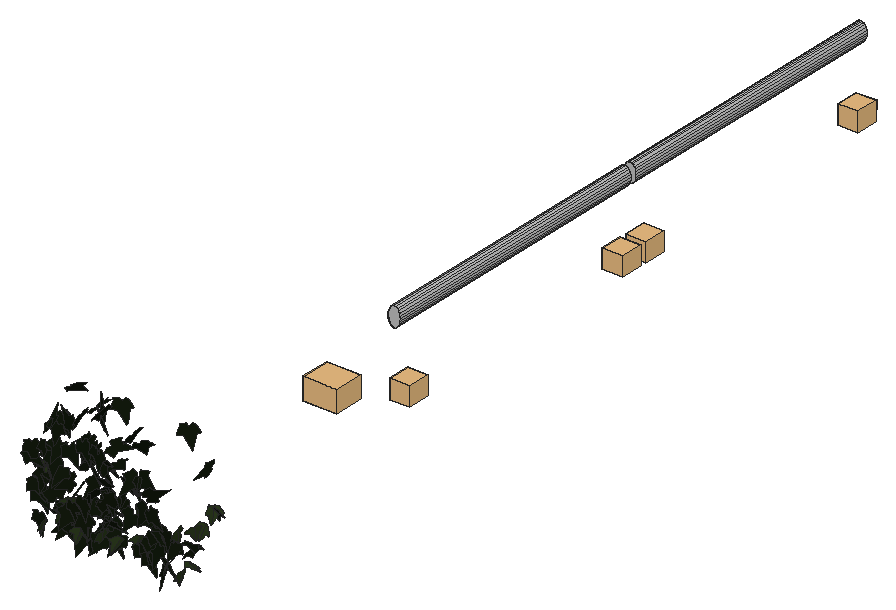
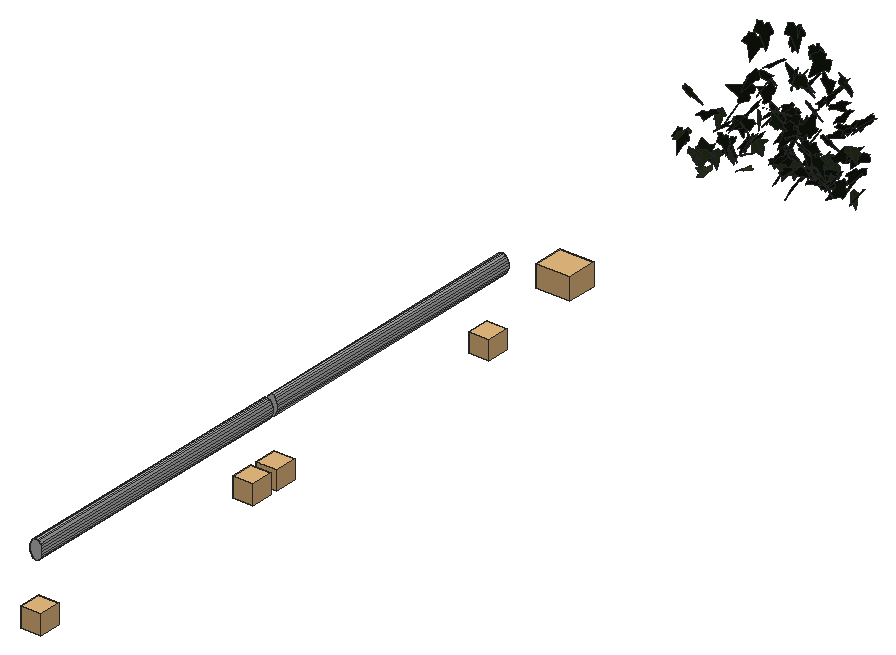
# SketchUp Ruby script. Lengths in inches.
U = 1.inch
M = Sketchup.active_model
def pt(a) = Geom::Point3d.new(a.map { |v| v * U })
def face(e, loops, mat)
  f = e.add_face(loops[0].map { |a| pt(a) })
  loops[1..].each { |l| e.add_face(l.map { |a| pt(a) }).erase! }
  f.material = f.back_material = mat if mat
  f
end
# faces: each face lists its corners as indices into pts; further lists are holes
def faces(e, pts, list, mat = nil) = list.each { |f| face(e, (f[0].is_a?(Array) ? f : [f]).map { |l| l.map { |i| pts[i] } }, mat) }
# xy, xz, yz: faces in a plane at the given z, y or x. An outline is a flat list of corners, or four numbers for a rectangle; further outlines are holes
def ring(l) = l.size == 4 ? [[l[0], l[1]], [l[2], l[1]], [l[2], l[3]], [l[0], l[3]]] : l.each_slice(2).to_a
def flat(e, list, mat, &to3) = list.each { |f| face(e, (f[0].is_a?(Array) ? f : [f]).map { |l| ring(l).map { |u, v| to3.(u, v) } }, mat) }
def xy(e, z, list, mat = nil) = flat(e, list, mat) { |x, y| [x, y, z] }
def xz(e, y, list, mat = nil) = flat(e, list, mat) { |x, z| [x, y, z] }
def yz(e, x, list, mat = nil) = flat(e, list, mat) { |y, z| [x, y, z] }
def lines(e, pts, list) = list.each { |a, b| e.add_line(pt(pts[a]), pt(pts[b])) }
# prism: a flat outline (further loops are holes) pulled along v
def prism(e, loops, v, mat = nil)
  f = face(e, loops, mat); d = Geom::Vector3d.new(v.map { |x| x * U })
  f.pushpull(f.normal.samedirection?(d) ? d.length : -d.length)
end
def box(e, o, s, mat = nil) = prism(e, [[o, [o[0] + s[0], o[1], o[2]], [o[0] + s[0], o[1] + s[1], o[2]], [o[0], o[1] + s[1], o[2]]]], [0, 0, s[2]], mat)
def at(x, y, z, deg = 0) = Geom::Transformation.translation(pt([x, y, z])) * Geom::Transformation.rotation(ORIGIN, Z_AXIS, deg.degrees)
def axes(o, x, y, z) = Geom::Transformation.new([*x, 0, *y, 0, *z, 0, *pt(o).to_a, 1])
def part(name) = M.definitions.add(name)
# library, detail: a bought-in or finely detailed component or shape, given as its bounding box
def library(name, o, s) = part(name).tap { |d| box(d.entities, o, s) }
def detail(e, o, s) = box(e.add_group.entities, o, s)
def put(e, d, t, mat = nil) = e.add_instance(d, t).tap { |i| i.material = mat if mat }
def group(e, t, mat = nil) = e.add_group.tap { |g| g.transformation = t; g.material = mat if mat }.entities
root = M.entities
M.materials.add("Glass Rail Metal").color = [192, 192, 192]
M.materials.add("[Translucent Glass Safety]").color = [204, 235, 244]
M.materials["[Translucent Glass Safety]"].alpha = 0.5
M.materials.add("[Translucent Glass Tinted]").color = [8, 201, 241]
M.materials["[Translucent Glass Tinted]"].alpha = 0.48
M.materials.add("efeu1").color = [18, 25, 13]
M.materials.add("efeu2").color = [43, 57, 29]
c1 = part("ivyleaf_9")
p = [[1.54,2.16,1.25],[1.36,2.04,1.19],[-0.21,0.99,0.68],[-0.71,1.11,0.82],[-0.85,0.86,0.67],[-0.8,0.17,0.21],
  [-0.9,-0.01,0.1],[-0.67,-0.16,-0.02],[-0.08,-0.08,-0.05],[-0.03,-0.6,-0.4],[0.65,-0.88,-0.66],[0.83,-0.6,-0.49],
  [1.29,-0.42,-0.43],[1.8125,-0.07,-0.26],[1.21,0.44,0.15]]
faces(c1.entities,p,[[0,1,2,3,4,5,6,7,8,9,10,11,12,13,14]],"efeu1")
c2 = part("ivyleaf_10")
p = [[0,0.5,-0.03],[-0.0625,2.02,-0.43],[-0.19,2.01,-0.46],[-0.54,1.05,-0.29],[-0.52,0.625,-0.18],[-0.83,0.76,-0.28],
  [-1.16,0.64,-0.33],[-1.15,0.33,-0.24],[-0.77,-0.39,0.02],[-0.3,-0.51,0.16],[0.04,-0.48,0.23],[-0.02,2.01,-0.4375],
  [-0.06,2.01,-0.43],[0.04,-0.49,0.23],[0.67,-0.49,0.14],[1.38,0.36,-0.2],[1.375,0.51,-0.24],[0.81,0.65,-0.19],
  [0.62,0.59,-0.15],[0.6,1.09,-0.28],[0.5,1.23,-0.31]]
faces(c2.entities,p,[[0,1,2,3,4,5,6,7,8,9,10],[11,12,0,13,14,15,16,17,18,19,20]],"efeu2")
c3 = library("glass bracket3\#1",[-0.84,-0.98,-1],[3.67,3.29,2])
c4 = library("Group\#37",[0,0,0],[3.67,3.3,2.01])
c5 = part("Group572\#1")
prism(c5.entities,[[[0.5,0,-0.87],[0.71,0,-0.71],[0.87,0,-0.5],[0.97,0,-0.26],[1,0,0],[0.97,0,0.26],[0.87,0,0.5],[0.71,0,0.71],[0.5,0,0.87],[0.26,0,0.97],[0,0,1],[-0.26,0,0.97],[-0.5,0,0.87],[-0.71,0,0.71],[-0.87,0,0.5],[-0.97,0,0.26],[-1,0,0],[-0.97,0,-0.26],[-0.87,0,-0.5],[-0.71,0,-0.71],[-0.5,0,-0.87],[-0.26,0,-0.97],[0,0,-1],[0.26,0,-0.97]]],[0,46.9,0],"Glass Rail Metal")
c6 = part("Group575\#2")
prism(c6.entities,[[[0.5,0,-0.87],[0.71,0,-0.71],[0.87,0,-0.5],[0.97,0,-0.26],[1,0,0],[0.97,0,0.26],[0.87,0,0.5],[0.71,0,0.71],[0.5,0,0.87],[0.26,0,0.97],[0,0,1],[-0.26,0,0.97],[-0.5,0,0.87],[-0.71,0,0.71],[-0.87,0,0.5],[-0.97,0,0.26],[-1,0,0],[-0.97,0,-0.26],[-0.87,0,-0.5],[-0.71,0,-0.71],[-0.5,0,-0.87],[-0.26,0,-0.97],[0,0,-1],[0.26,0,-0.97]]],[0,46.9,0],"Glass Rail Metal")
put(root,c1,axes([575.92,120.95,317.45],[0.67615,-0.93162,-0.66201],[0.05924,0.79673,-1.0607],[1.14135,0.51055,0.44724]))
put(root,c1,axes([583.66,122.125,308.17],[-0.57165,-1.06868,0.43413],[-0.12193,-0.42582,-1.20878],[1.14704,-0.57786,0.08786]))
put(root,c1,axes([580.53,121.9,317.56],[-0.13213,-1.30218,0.02339],[-0.00565,-0.02293,-1.30886],[1.30238,-0.13221,-0.00331]))
put(root,c1,axes([602.59,121.65,308.34],[-1.09508,-0.1847,-0.62254],[0.60794,0.13734,-1.11015],[0.22821,-1.25216,-0.02993]))
put(root,c1,axes([597.58,121.83,319.51],[-1.25599,-0.35142,0.02931],[-0.02481,-0.02008,-1.30416],[0.35177,-1.25617,0.01265]))
put(root,c1,axes([591.37,121.375,326.84],[0.52135,-0.86623,0.94791],[-0.32482,0.90082,1.00185],[-1.24233,-0.59905,0.13585]))
put(root,c1,axes([592.03,120.58,314.14],[0.1064,-0.07283,-1.33171],[0.02502,1.33581,-0.07105],[1.33346,-0.01925,0.10759]))
put(root,c1,axes([587.91,122.33,304.16],[0.04589,-0.86139,0.97001],[0.25591,-0.94553,-0.85176],[1.27177,0.22135,0.13639]))
put(root,c1,axes([586.4,122.09,311.1875],[0.32129,-1.2243,0.35256],[0.08289,-0.34274,-1.26574],[1.27135,0.33175,-0.00658]))
put(root,c1,axes([586.62,121.26,327.66],[-0.48913,1.20004,-0.36765],[0.18426,-0.32165,-1.29503],[-1.24149,-0.52054,-0.04735]))
put(root,c1,axes([596.4,122.47,311.93],[-0.42387,-1.07127,0.62758],[0.00682,-0.66514,-1.13079],[1.24155,-0.36209,0.22047]))
put(root,c1,axes([589.35,122.27,321.37],[0.19565,-1.25727,0.37387],[0.08967,-0.3643,-1.27201],[1.30861,0.21294,0.03127]))
put(root,c1,axes([586.6875,121.8,322.2],[0.40295,-1.21226,-0.24904],[-0.0505,0.24558,-1.27715],[1.23654,0.40507,0.029]))
put(root,c1,axes([591.04,121.02,329.89],[-0.13439,1.3952,-0.04116],[0.00983,-0.04041,-1.40165],[-1.39578,-0.13462,-0.00591]))
put(root,c1,axes([597.57,121,327.97],[-0.17355,1.39179,0.02506],[-0.00251,0.02494,-1.40256],[-1.39201,-0.17357,-0.00059]))
put(root,c1,axes([575.92,121.96,318.43],[0.08834,-1.26485,-0.32961],[-0.0691,0.32538,-1.26714],[1.30527,0.10283,-0.04477]))
put(root,c2,axes([585.81,122.1,305.67],[-0.48165,-1.05232,0.44016],[0.12129,-0.52233,-1.11605],[1.1342,-0.39102,0.30627]))
put(root,c1,axes([580.63,122.57,323.14],[-0.07599,-1.23712,0.38307],[0.05682,-0.38655,-1.23707],[1.29383,-0.05569,0.07683]))
put(root,c1,axes([600.83,121.61,314.41],[0.74121,-0.91425,-0.59007],[-0.24816,0.55312,-1.16873],[1.05946,0.76918,0.13907]))
put(root,c1,axes([600.27,121.95,306],[0.34478,-1.19798,-0.46052],[-0.10615,0.4486,-1.24644],[1.27905,0.36016,0.02069]))
put(root,c1,axes([598.55,121.79,307.15],[0.5325,-1.0837,-0.55234],[0.00066,0.60321,-1.18287],[1.21634,0.47411,0.24245]))
put(root,c1,axes([599.71,122.73,305.36],[0.02652,-0.58453,1.12018],[0.26568,-1.0928,-0.57653],[1.23527,0.24758,0.09995]))
put(root,c1,axes([591.6,122.26,314.125],[0.21702,-1.24933,-0.14827],[0.06594,0.16155,-1.2647],[1.25637,0.20732,0.09199]))
put(root,c1,axes([586.61,122.43,307.82],[0.10516,-1.30888,-0.29519],[-0.04501,0.29249,-1.31293],[1.341,0.11246,-0.02092]))
put(root,c1,axes([589.22,122.2,321.4375],[-1.09356,0.72884,-0.16345],[0.02609,-0.25235,-1.29979],[-0.74649,-1.07653,0.19402]))
put(root,c1,axes([581.125,122.8,319.82],[-0.73536,-1.04333,0.06805],[-0.01687,-0.07135,-1.27614],[1.04541,-0.73504,0.02728]))
put(root,c1,axes([585.8125,122.89,304.02],[-0.68303,-1.03968,0.03527],[0.14021,-0.13382,-1.22929],[1.03079,-0.67072,0.19059]))
put(root,c1,axes([600.78,121.65,309.51],[0.21311,-0.46274,-1.28453],[0.4518,1.25074,-0.37561],[1.28841,-0.36205,0.34418]))
put(root,c1,axes([583.42,122.34,320.05],[0.22533,-1.16194,-0.53232],[0.08295,0.55268,-1.17128],[1.27538,0.16934,0.17023]))
put(root,c1,axes([576.72,122.29,311.73],[-0.26944,-0.92664,-0.92044],[0.40606,0.83381,-0.9583],[1.24136,-0.47387,0.11368]))
put(root,c1,axes([594.66,122.46,314.58],[-1.05561,0.65223,-0.3732],[0.29046,-0.23936,-1.23989],[-0.69304,-1.09375,0.04879]))
put(root,c1,axes([580.04,121.36,323.46],[-1.01888,0.94532,-0.49777],[-0.36606,0.33731,1.38987],[1.00369,1.08265,0.0016]))
put(root,c2,axes([587.31,122.16,305.98],[0.70732,-0.94028,-0.41999],[0.02741,0.52652,-1.13262],[1.02945,0.63204,0.31873]))
put(root,c2,axes([577.8,122.56,303.93],[0.28354,-1.20234,0.01427],[0.00088,-0.01445,-1.23532],[1.20242,0.28353,-0.00246]))
put(root,c1,axes([602.71,122.95,304.05],[-0.67486,-0.00221,-1.0844],[1.05058,-0.31785,-0.65316],[-0.26873,-1.23707,0.16976]))
put(root,c1,axes([589.45,123.29,304.82],[-0.84809,-0.90696,0.2864],[-0.02112,-0.36567,-1.22053],[0.95087,-0.81705,0.22833]))
put(root,c1,axes([588.02,122.85,322.41],[-1.14494,0.21205,-0.56374],[0.52647,-0.23585,-1.15795],[-0.29257,-1.25422,0.12243]))
put(root,c1,axes([594.81,122.87,316.9],[0.62865,-0.57449,0.99092],[0.73389,-0.66583,-0.8516],[0.87941,0.96633,0.00232]))
put(root,c2,axes([593.0625,123.17,305.66],[-0.45559,-0.84555,0.79662],[0.01286,-0.85931,-0.90473],[1.16163,-0.32211,0.32245]))
put(root,c1,axes([600.86,122.21,310.28],[0.73325,-0.84139,-0.73851],[-0.17637,0.78497,-1.06944],[1.10555,0.68328,0.31921]))
put(root,c1,axes([598.33,123.62,313.125],[-0.23159,-1.06441,0.75246],[-0.09193,-0.749,-1.08781],[1.30027,-0.24254,0.0571]))
put(root,c1,axes([590.32,122.07,312.19],[1.21473,0.3756,-0.03514],[-0.03345,-0.01078,-1.27148],[-0.37575,1.21519,-0.00042]))
put(root,c1,axes([598.77,122.87,306.8125],[0.52928,-1.17601,-0.19376],[-0.06183,0.18463,-1.28949],[1.19026,0.53254,0.01918]))
put(root,c1,axes([582.98,122.94,305.15],[-0.01894,0.0737,-1.25395],[-0.83171,-0.94053,-0.04272],[-0.94131,0.82954,0.06297]))
put(root,c2,axes([581.73,122.07,307.43],[-0.07706,-0.87526,-0.91098],[0.27949,0.87825,-0.86745],[1.23201,-0.25398,0.13981]))
put(root,c1,axes([580.92,123.61,314.73],[-0.67514,-1.0514,0.26656],[-0.04197,-0.28842,-1.24393],[1.08385,-0.66609,0.11787]))
put(root,c1,axes([583.27,123.34,308.9],[0.41083,-1.15155,0.26388],[0.09727,-0.24546,-1.22261],[1.17739,0.42209,0.00893]))
put(root,c1,axes([576.33,123.33,304.57],[0.30529,-1.2282,0.10539],[0.01737,-0.10428,-1.26555],[1.23259,0.30568,-0.00826]))
put(root,c1,axes([576.99,123.65,312.4],[-0.11687,-1.20869,0.31111],[-0.07131,-0.3055,-1.21366],[1.24605,-0.13085,-0.04027]))
put(root,c1,axes([598.25,122.28,325.98],[0.80015,1.02322,-0.25314],[-0.17804,-0.18204,-1.29863],[-1.03892,0.81925,0.02759]))
put(root,c1,axes([602.73,123.66,310.3],[0.23182,-1.144,0.52617],[0.08839,-0.51891,-1.16716],[1.2561,0.24765,-0.01498]))
put(root,c1,axes([595.85,123.19,318.14],[0.57248,-1.16183,-0.0931],[-0.04645,0.08091,-1.2952],[1.16463,0.57433,-0.00589]))
put(root,c1,axes([580.3,122.72,309.69],[-1.0841,-0.6406,0.46027],[0.40928,0.21196,1.25899],[-0.67432,1.15853,0.02417]))
put(root,c1,axes([593.92,123.03,313.49],[0.79333,-1.01362,-0.28741],[-0.0764,0.30348,-1.2812],[1.05081,0.78732,0.12383]))
put(root,c1,axes([598.06,122.41,319.64],[0.43241,-0.61036,-1.13884],[-0.34907,1.10108,-0.72267],[1.24405,0.52111,0.19306]))
put(root,c1,axes([592.81,123.74,306.03],[-0.92375,-0.92692,0.09963],[-0.06637,-0.0745,-1.30861],[0.92989,-0.92611,0.00556]))
put(root,c2,axes([589.66,123.03,305.78],[-0.01694,-1.25629,-0.14216],[0.11707,0.14,-1.25118],[1.25888,-0.02992,0.11444]))
put(root,c2,axes([582.67,123.5,309.43],[-0.51007,-1.02092,0.52289],[-0.14253,-0.51141,-1.13754],[1.13815,-0.52158,0.09188]))
put(root,c2,axes([596.9375,123.59,307.24],[-0.38,-1.07178,0.54613],[0.04991,-0.58629,-1.11586],[1.20187,-0.31452,0.21902]))
put(root,c1,axes([590.26,122.58,311.62],[1.26306,0.22876,0.34521],[0.34264,0.04508,-1.28351],[-0.2326,1.30861,-0.01613]))
put(root,c1,axes([582.29,123.95,304.88],[-0.94126,-0.79553,0.25258],[-0.0857,-0.28657,-1.22195],[0.83025,-0.93148,0.16022]))
put(root,c1,axes([602.47,123.43,305.04],[0.94866,-0.8233,0.11988],[0.08545,-0.08443,-1.25607],[0.82758,0.95247,-0.00773]))
put(root,c1,axes([576.29,123.3,309.31],[0.05158,-1.01345,-0.78375],[0.12578,0.7846,-1.00627],[1.27496,-0.0364,0.13098]))
put(root,c1,axes([582.98,123.51,313.1],[-1.18141,0.30894,0.32486],[-0.31338,0.08569,-1.22114],[-0.32059,-1.22227,-0.0035]))
put(root,c1,axes([578.61,123.92,317.14],[-0.82465,-0.82912,-0.47806],[0.49122,0.17492,-1.15071],[0.82139,-0.93701,0.20821]))
put(root,c1,axes([588.9,123.2,313.61],[-0.06046,1.1603,-0.56671],[-0.35209,-0.56065,-1.11032],[-1.24237,0.10242,0.34225]))
put(root,c1,axes([590.56,123.63,308.6],[-1.06256,0.63676,-0.30987],[0.15289,-0.33928,-1.22149],[-0.69146,-1.05353,0.20608]))
put(root,c2,axes([602.45,123.8125,303.88],[0.65827,-0.99824,0.31042],[0.16257,-0.26462,-1.19571],[1.03267,0.67798,-0.00964]))
put(root,c1,axes([604.06,124.38,308.27],[-0.48348,-1.06031,0.46299],[0.04857,-0.51994,-1.14002],[1.15596,-0.42163,0.24154]))
put(root,c1,axes([577.2,124.17,317.56],[0.0071,-1.25666,0.16762],[-0.03638,-0.16776,-1.25614],[1.26727,0.00222,-0.037]))
put(root,c1,axes([581.95,124.25,307.64],[-0.97037,-0.78716,0.04801],[0.06403,-0.15452,-1.23918],[0.78602,-0.95919,0.16022]))
put(root,c2,axes([596.89,123.33,312.71],[0.83894,-0.77947,-0.52171],[-0.15845,0.57212,-1.10957],[0.92447,0.8054,0.28327]))
put(root,c1,axes([599.05,123.32,315.8125],[0.36792,-0.11223,1.30728],[1.29042,0.27669,-0.33942],[-0.23748,1.32959,0.18098]))
put(root,c1,axes([603.94,123.4375,305.875],[-0.35907,1.18933,0.13807],[-0.05902,0.12639,-1.24219],[-1.19586,-0.36334,0.01985]))
put(root,c1,axes([582.53,123.59,323.1],[0.1049,-0.10865,1.36057],[-0.78396,1.11225,0.14927],[-1.1173,-0.79062,0.02301]))
put(root,c1,axes([580.02,124.59,307.08],[0.25054,-1.21851,0.13044],[0.01664,-0.12975,-1.24396],[1.22536,0.2509,-0.00977]))
put(root,c1,axes([575.91,124.43,308.16],[0.37678,-1.19637,-0.10522],[0.01359,0.11451,-1.25341],[1.20091,0.37406,0.04719]))
put(root,c1,axes([589.17,123.58,315.3125],[1.22836,0.21743,-0.26564],[-0.2777,0.04919,-1.24385],[-0.2018,1.25579,0.09472]))
put(root,c1,axes([590.15,123.71,307.61],[1.16548,0.13479,0.4986],[0.49231,0.08229,-1.17302],[-0.15621,1.26498,0.02318]))
put(root,c1,axes([584.48,124.4,307.15],[-1.075,0.5842,-0.24994],[0.17196,-0.20539,-1.21968],[-0.61171,-1.08439,0.09636]))
put(root,c1,axes([585.9,123.66,310.91],[0.15004,1.27275,-0.06793],[-0.0056,-0.06774,-1.28156],[-1.27455,0.15012,-0.00236]))
put(root,c2,axes([576.63,124.44,313.68],[1.22008,0.04788,-0.28919],[-0.29082,0.04286,-1.21988],[-0.03667,1.25315,0.05277]))
put(root,c2,axes([604.41,124.27,310.84],[-0.00323,-1.20526,-0.37549],[0.05285,0.37503,-1.20425],[1.26129,-0.0188,0.0495]))
put(root,c1,axes([589.87,125.29,305.46],[-1.03565,-0.55013,0.4761],[-0.3843,-0.28961,-1.1706],[0.61776,-1.10243,0.06994]))
put(root,c1,axes([582.93,124.18,305.82],[-0.76947,0.89212,0.46128],[-0.3322,0.32231,-1.1775],[-0.94779,-0.83724,0.03822]))
put(root,c2,axes([604.875,124.65,303.02],[0.07674,-1.24687,-0.06836],[-0.00234,0.06835,-1.24923],[1.24874,0.07676,0.00186]))
put(root,c2,axes([590.36,124.43,305.78],[-1.24869,0.20497,-0.02115],[0.01215,-0.05646,-1.26426],[-0.2057,-1.2476,0.05374]))
put(root,c1,axes([590.42,124.94,307.7],[-0.00761,-1.24236,-0.31069],[-0.01718,0.31077,-1.24224],[1.2805,-0.00321,-0.01851]))
put(root,c1,axes([578.51,124.09,305.79],[1.23228,-0.00824,0.08599],[0.08569,0.27253,-1.20181],[-0.01096,1.20484,0.27243]))
put(root,c1,axes([590.72,124.99,304.61],[0.75577,-0.99232,-0.24267],[-0.18588,0.16325,-1.24643],[1.00451,0.77681,-0.04806]))
put(root,c1,axes([579.69,125.33,323.48],[0.32323,-1.24208,-0.36903],[-0.07095,0.3628,-1.28326],[1.29379,0.3302,0.02182]))
put(root,c1,axes([585.24,126.13,315.16],[0.55284,-0.9066,0.83292],[0.41013,-0.72528,-1.06164],[1.16081,0.68802,-0.02159]))
put(root,c1,axes([584.29,125.97,320.04],[-1.19779,0.42356,-0.31129],[0.25861,-0.19955,-1.26661],[-0.45763,-1.22138,0.09899]))
put(root,c1,axes([584.04,126.71,315.21],[0.38475,0.62265,1.21882],[-0.97871,-0.75985,0.69714],[0.95673,-1.02771,0.223]))
put(root,c1,axes([582.59,125.94,310.48],[-0.61647,1.12045,-0.04647],[0.01395,-0.04537,-1.27881],[-1.12133,-0.61655,0.00964]))
put(root,c1,axes([585.37,126.73,312.39],[-1.23392,-0.03464,-0.33159],[0.3334,-0.12532,-1.22754],[0.00076,-1.27154,0.13001]))
put(root,c1,axes([585.49,126.96,307.77],[-1.11368,-0.49067,0.33093],[-0.30608,-0.12605,-1.21696],[0.50654,-1.15495,-0.00777]))
put(root,c1,axes([585.47,126.88,308.03],[-1.19226,-0.39882,0.11055],[-0.10119,-0.04599,-1.25714],[0.4013,-1.19649,0.01147]))
put(root,c2,axes([597.13,127.3,304.01],[-1.15628,-0.15894,0.42271],[0.19623,-1.22332,0.07681],[0.40674,0.13837,1.16462]))
put(root,c1,axes([581.42,125.54,329.38],[0.9247,0.90864,0.36879],[0.15306,0.36694,-1.28788],[-0.96861,0.92543,0.14856]))
put(root,c1,axes([585.69,128.56,315.08],[-0.34849,-1.19969,0.60049],[0.65213,-0.69367,-1.00739],[1.17242,0.02925,0.73883]))
put(root,c1,axes([594.33,128.03,308.5],[0.5442,-1.11221,-0.34276],[0.57383,0.58561,-0.98915],[1.01252,0.2659,0.74481]))
put(root,c1,axes([586.12,127.67,324.23],[0.04593,-0.81568,1.1596],[0.10189,1.1591,0.81129],[-1.41408,0.05702,0.09612]))
put(root,c1,axes([603.82,128.9,305.18],[-0.28099,-1.14493,-0.38615],[1.20815,-0.26009,-0.10798],[0.0187,-0.40053,1.17395]))
put(root,c1,axes([588.01,128.9375,315.83],[0.03342,-1.2785,-0.16921],[1.25862,0.06925,-0.27458],[0.28119,-0.15797,1.24912]))
put(root,c1,axes([603.73,129.18,306.01],[-0.31053,-1.08358,0.52383],[0.86888,-0.57618,-0.67678],[0.83281,0.1971,0.90141]))
put(root,c1,axes([589.05,129.03,327.57],[-0.0399,-1.36407,-0.18827],[0.39925,0.1688,-1.30761],[1.31785,-0.09243,0.39045]))
put(root,c1,axes([584.04,128.7,325.22],[0.50089,-1.32792,0.33],[1.34101,0.54625,0.16268],[-0.27197,0.24778,1.4099]))
put(root,c1,axes([584.87,128.44,314.93],[1.03092,-0.88323,-0.41558],[-0.31599,0.26993,-1.35753],[0.92356,1.07826,-0.00058]))
put(root,c1,axes([586.07,128.125,315.71],[1.36524,0.11763,-0.26031],[-0.26065,-0.00713,-1.37021],[-0.11688,1.38982,0.015]))
put(root,c2,axes([603.25,129.08,302.27],[-0.27921,-1.11082,0.44805],[1.19777,-0.25743,0.10818],[-0.00393,0.46091,1.14025]))
put(root,c1,axes([584.7,128.97,306.35],[0.71194,-1.08577,-0.48085],[-0.25244,0.40946,-1.29831],[1.16034,0.75527,0.01258]))
put(root,c1,axes([587.02,128.98,318.76],[0.93543,-0.82079,-0.37371],[0.76738,1.00726,-0.29145],[0.4738,-0.01088,1.20987]))
put(root,c2,axes([602.125,131.71,307.26],[-0.77059,-0.97621,-0.09235],[0.06148,0.06912,-1.24369],[0.97864,-0.77302,0.00542]))
put(root,c2,axes([603.1875,132.51,307.64],[1.21498,-0.16921,-0.23175],[-0.22513,0.06304,-1.22632],[0.17792,1.23527,0.03084]))
put(root,c1,axes([604.37,132.67,319.07],[-1.13239,0.59359,-0.16592],[0.02297,-0.30619,-1.25216],[-0.61591,-1.10277,0.25836]))
put(root,c2,axes([604.57,133.47,311.04],[0.61172,1.06216,-0.2768],[-0.14432,-0.23631,-1.2257],[-1.08811,0.62848,0.00695]))
put(root,c1,axes([604.53,133.51,311.0625],[1.01,0.35121,-0.65953],[-0.67366,-0.05178,-1.05921],[-0.32328,1.20515,0.14669]))
put(root,c1,axes([595.1,138.86,320.65],[-0.32135,-1.15058,-0.4979],[0.4022,0.39221,-1.16593],[1.18742,-0.44423,0.26018]))
put(root,c3,axes([590.29,178.46,309.14],[1.9,0,0],[0,1.9,0],[0,0,2.261]),"[Translucent Glass Tinted]")
put(root,c4,axes([597.22,193.77,301.06],[0,1.28,0],[-1.28,0,0],[0,0,1.99144]),"[Translucent Glass Safety]")
put(root,c5,axes([593.9375,193.75,316.8125],[1.28,0,0],[0,1.28,0],[0,0,1.99144]))
put(root,c4,axes([597.22,253.79,305.06],[0,-1.28,0.00027],[-1.28,0,0],[0,-0.00017,-1.99144]),"[Translucent Glass Safety]")
put(root,c4,axes([597.22,255.21,301.06],[0,1.28,0],[-1.28,0,0],[0,0,1.99144]),"[Translucent Glass Safety]")
put(root,c6,axes([593.9375,255.19,316.8125],[1.28,0,0],[0,1.28,0],[0,0,1.99144]))
put(root,c4,axes([597.22,315.23,305.06],[0,-1.28,0.00027],[-1.28,0,0],[0,-0.00017,-1.99144]),"[Translucent Glass Safety]")
